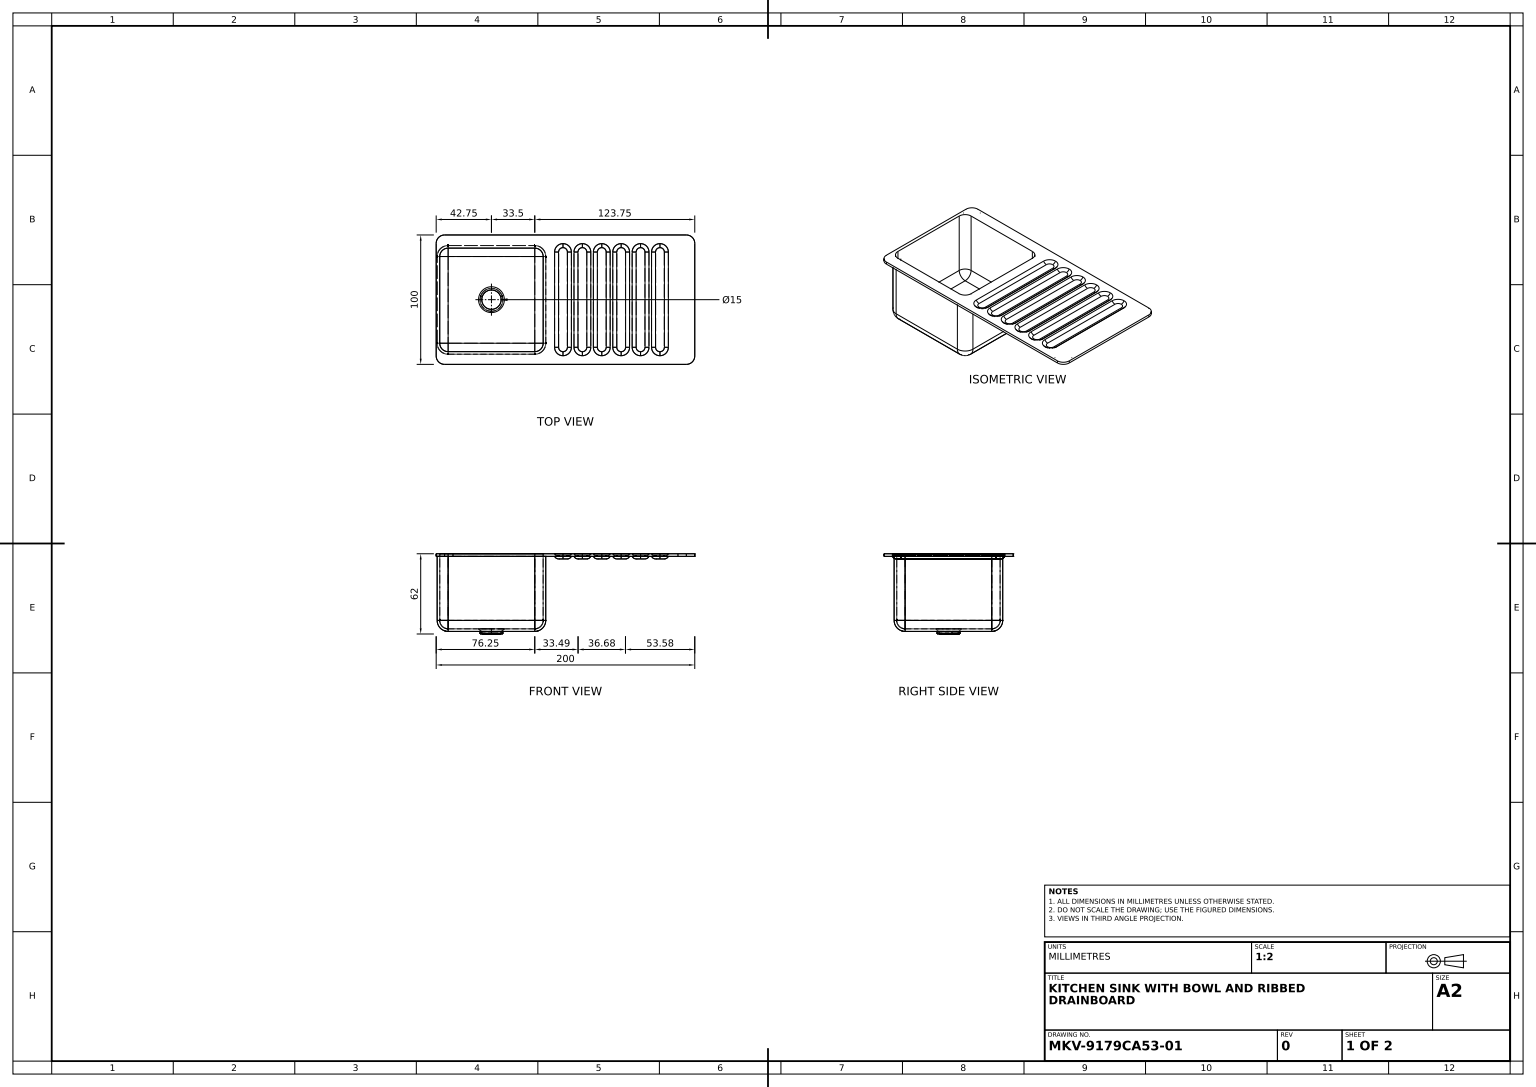
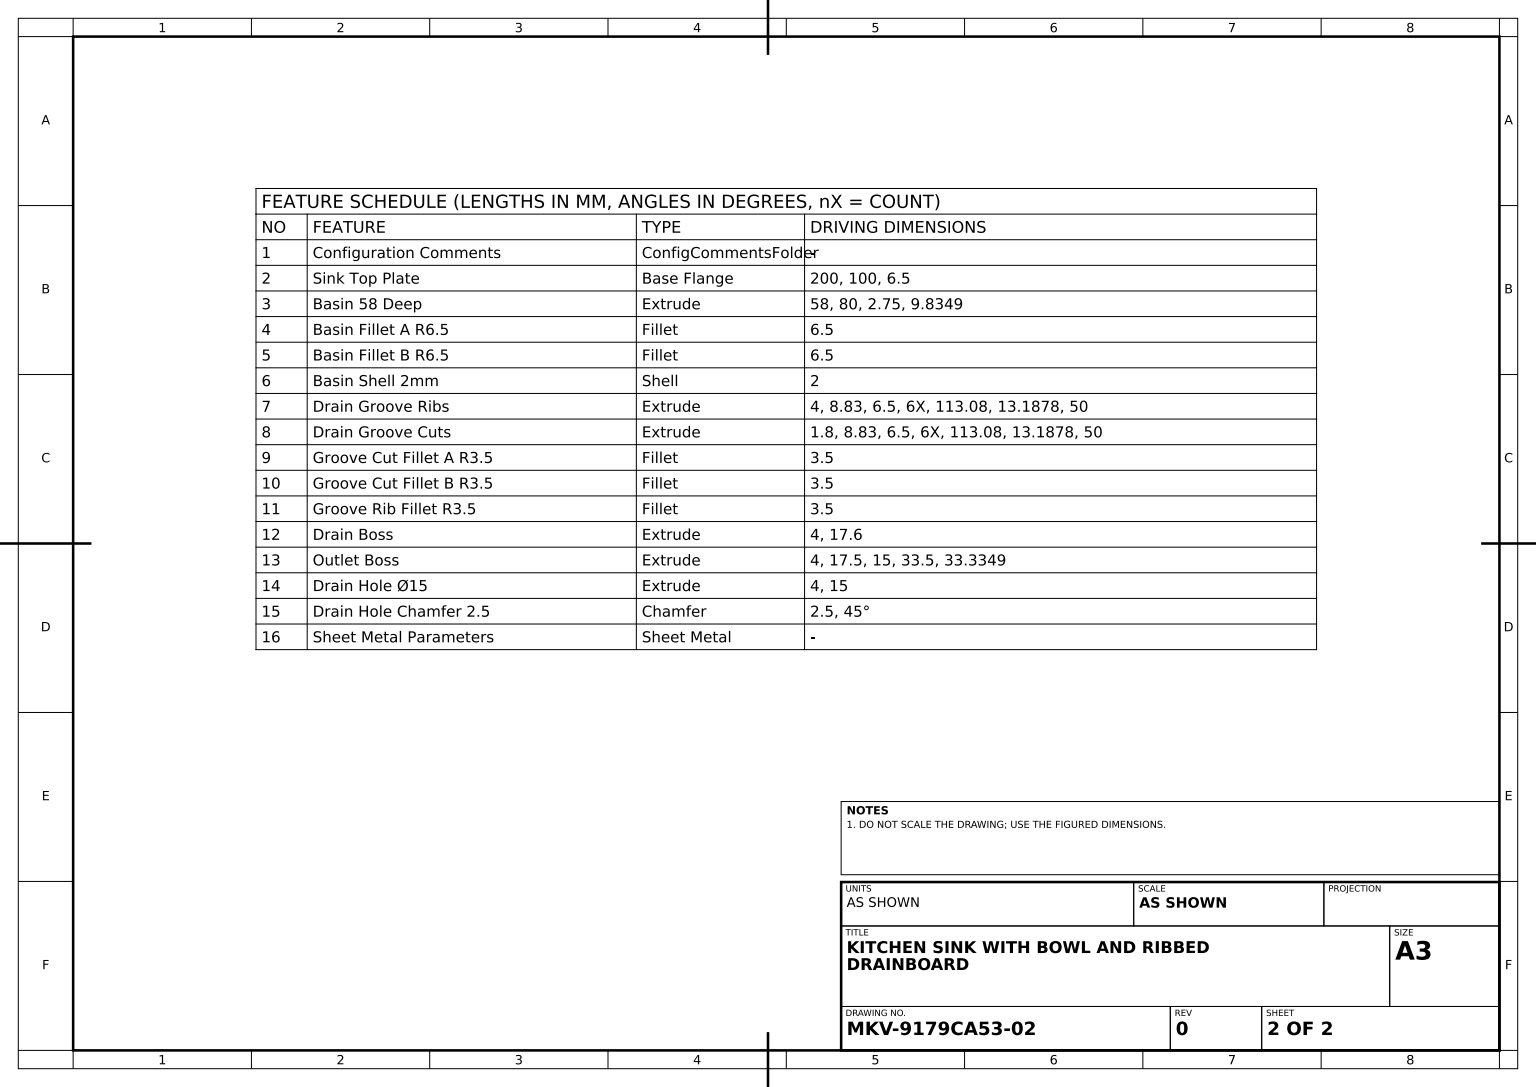
solid
v1 (16.520588,-1.8,36.8122)
v2 (19.58,0,36.8122)
e1 v1 v2 CIRCLE(AX(P(16.520588,1.7,36.8122),D(0,0,1),D(1,0,0)),3.5)
v3 (13.08,-1.8,40.252788)
e2 v3 v1 CIRCLE(AX(P(13.08,-1.8,36.8122),D(0,1,0),D(0,0,1)),3.440588)
v4 (13.08,0,43.3122)
e3 v4 v3 CIRCLE(AX(P(13.08,1.7,40.252788),D(1,0,0),D(0,0,-1)),3.5)
e4 v4 v2 CIRCLE(AX(P(13.08,0,36.8122),D(0,1,0),D(0,0,1)),6.5)
face TORUS(AX(P(13.08,1.7,36.8122),D(0,-1,0),D(0,0,-1)),3.440588,3.5) rev [-e1 -e2 -e3 e4]
v5 (9.742278,-4,36.8122)
v6 (6.58,-2,36.8122)
e5 v5 v6 CIRCLE(AX(P(9.742278,-0.5,36.8122),D(0,0,-1),D(-1,0,0)),3.5)
v7 (13.08,-4,40.149922)
e6 v7 v5 CIRCLE(AX(P(13.08,-4,36.8122),D(0,-1,0),D(0,0,1)),3.337722)
v8 (13.08,-2,43.3122)
e7 v8 v7 CIRCLE(AX(P(13.08,-0.5,40.149922),D(1,0,0),D(0,0,-1)),3.5)
e8 v8 v6 CIRCLE(AX(P(13.08,-2,36.8122),D(0,-1,0),D(0,0,-1)),6.5)
face TORUS(AX(P(13.08,-0.5,36.8122),D(0,-1,0),D(0,0,-1)),3.337722,3.5) [-e5 -e6 -e7 e8]
v9 (-90.75,-60,33.665098)
v10 (-23.75,-60,33.665098)
e9 v9 v10 LINE
v11 (-90.75,-60,-33.334902)
e10 v11 v9 LINE
v12 (-23.75,-60,-33.334902)
e11 v12 v11 LINE
e12 v10 v12 LINE
v13 (-48.887462,-60,-2.574969)
v14 (-57.25,-60,8.965098)
e13 v13 v14 CIRCLE(AX(P(-57.25,-60,0.165098),D(0,-1,0),D(0,0,-1)),8.8)
v15 (-65.612538,-60,-2.574969)
e14 v15 v13 CIRCLE(AX(P(-57.25,-60,0),D(0,-1,0),D(0,0,-1)),8.75)
e15 v14 v15 CIRCLE(AX(P(-57.25,-60,0.165098),D(0,-1,0),D(0,0,-1)),8.8)
face PLANE(AX(P(0,-60,0),D(0,-1,0),D(0,0,-1))) [-e9 -e10 -e11 -e12] [-e13 -e14 -e15]
v16 (-1.92,-1.8,40.252788)
v17 (1.520588,-1.8,36.8122)
e16 v16 v17 CIRCLE(AX(P(-1.92,-1.8,36.8122),D(0,1,0),D(0,0,1)),3.440588)
v18 (1.520588,-1.8,-36.8122)
e17 v17 v18 LINE
v19 (-1.92,-1.8,-40.252788)
e18 v18 v19 CIRCLE(AX(P(-1.92,-1.8,-36.8122),D(0,1,0),D(0,0,1)),3.440588)
v20 (-5.360588,-1.8,-36.8122)
e19 v19 v20 CIRCLE(AX(P(-1.92,-1.8,-36.8122),D(0,1,0),D(0,0,1)),3.440588)
v21 (-5.360588,-1.8,36.8122)
e20 v20 v21 LINE
e21 v21 v16 CIRCLE(AX(P(-1.92,-1.8,36.8122),D(0,1,0),D(0,0,1)),3.440588)
face PLANE(AX(P(-1.92,-1.8,-36.8122),D(0,1,0),D(0,0,1))) [e16 e17 e18 e19 e20 e21]
v22 (9.639412,-1.8,-36.8122)
v23 (9.639412,-1.8,36.8122)
e22 v22 v23 LINE
v24 (6.58,0,-36.8122)
e23 v24 v22 CIRCLE(AX(P(9.639412,1.7,-36.8122),D(0,0,1),D(1,0,0)),3.5)
v25 (6.58,0,36.8122)
e24 v24 v25 LINE
e25 v23 v25 CIRCLE(AX(P(9.639412,1.7,36.8122),D(0,0,-1),D(-1,0,0)),3.5)
face CYL(AX(P(9.639412,1.7,-36.8122),D(0,0,1),D(1,0,0)),3.5) rev [-e22 -e23 e24 -e25]
v26 (58.08,0,-43.3122)
v27 (58.08,-1.8,-40.252788)
e26 v26 v27 CIRCLE(AX(P(58.08,1.7,-40.252788),D(-1,0,0),D(0,0,1)),3.5)
v28 (51.58,0,-36.8122)
e27 v26 v28 CIRCLE(AX(P(58.08,0,-36.8122),D(0,1,0),D(0,0,1)),6.5)
v29 (54.639412,-1.8,-36.8122)
e28 v28 v29 CIRCLE(AX(P(54.639412,1.7,-36.8122),D(0,0,1),D(1,0,0)),3.5)
e29 v27 v29 CIRCLE(AX(P(58.08,-1.8,-36.8122),D(0,1,0),D(0,0,1)),3.440588)
face TORUS(AX(P(58.08,1.7,-36.8122),D(0,-1,0),D(0,0,-1)),3.440588,3.5) rev [-e26 e27 e28 -e29]
v30 (61.417722,-4,-36.8122)
v31 (61.417722,-4,36.8122)
e30 v30 v31 LINE
v32 (58.08,-4,40.149922)
e31 v31 v32 CIRCLE(AX(P(58.08,-4,36.8122),D(0,-1,0),D(0,0,1)),3.337722)
v33 (54.742278,-4,36.8122)
e32 v32 v33 CIRCLE(AX(P(58.08,-4,36.8122),D(0,-1,0),D(0,0,1)),3.337722)
v34 (54.742278,-4,-36.8122)
e33 v33 v34 LINE
v35 (58.08,-4,-40.149922)
e34 v34 v35 CIRCLE(AX(P(58.08,-4,-36.8122),D(0,-1,0),D(0,0,1)),3.337722)
e35 v35 v30 CIRCLE(AX(P(58.08,-4,-36.8122),D(0,-1,0),D(0,0,1)),3.337722)
face PLANE(AX(P(58.08,-4,-36.8122),D(0,1,0),D(0,0,1))) rev [e30 e31 e32 e33 e34 e35]
v36 (-93.5,0,-50)
v37 (-100,0,-43.5)
e36 v36 v37 CIRCLE(AX(P(-93.5,0,-43.5),D(0,1,0),D(0,0,-1)),6.5)
v38 (-93.5,-2,-50)
e37 v38 v36 LINE
v39 (-100,-2,-43.5)
e38 v38 v39 CIRCLE(AX(P(-93.5,-2,-43.5),D(0,1,0),D(0,0,-1)),6.5)
e39 v39 v37 LINE
face CYL(AX(P(-93.5,-60,-43.5),D(0,1,0),D(0,0,1)),6.5) [-e36 -e37 e38 e39]
v40 (51.58,0,36.8122)
v41 (58.08,0,43.3122)
e40 v40 v41 CIRCLE(AX(P(58.08,0,36.8122),D(0,1,0),D(0,0,1)),6.5)
v42 (58.08,-1.8,40.252788)
e41 v41 v42 CIRCLE(AX(P(58.08,1.7,40.252788),D(1,0,0),D(0,0,-1)),3.5)
v43 (54.639412,-1.8,36.8122)
e42 v43 v42 CIRCLE(AX(P(58.08,-1.8,36.8122),D(0,1,0),D(0,0,1)),3.440588)
e43 v43 v40 CIRCLE(AX(P(54.639412,1.7,36.8122),D(0,0,-1),D(-1,0,0)),3.5)
face TORUS(AX(P(58.08,1.7,36.8122),D(0,-1,0),D(0,0,-1)),3.440588,3.5) rev [e40 e41 -e42 e43]
v44 (-17.25,-51.5,33.665098)
v45 (-17.25,0,33.665098)
e44 v44 v45 LINE
v46 (-23.75,-51.5,40.165098)
e45 v46 v44 CIRCLE(AX(P(-23.75,-51.5,33.665098),D(0,1,0),D(0,0,1)),6.5)
v47 (-23.75,0,40.165098)
e46 v47 v46 LINE
e47 v45 v47 CIRCLE(AX(P(-23.75,0,33.665098),D(0,-1,0),D(0,0,-1)),6.5)
face CYL(AX(P(-23.75,-58,33.665098),D(0,-1,0),D(0,0,-1)),6.5) rev [-e44 -e45 -e46 -e47]
v48 (6.58,-2,-36.8122)
v49 (9.742278,-4,-36.8122)
e48 v48 v49 CIRCLE(AX(P(9.742278,-0.5,-36.8122),D(0,0,1),D(1,0,0)),3.5)
e49 v5 v49 LINE
e50 v6 v48 LINE
face CYL(AX(P(9.742278,-0.5,-36.8122),D(0,0,1),D(1,0,0)),3.5) [e48 -e49 e5 e50]
v50 (-15.25,-2,33.665098)
v51 (-15.25,-2,-33.334902)
e51 v50 v51 LINE
v52 (-15.25,-51.5,33.665098)
e52 v52 v50 LINE
v53 (-15.25,-51.5,-33.334902)
e53 v53 v52 LINE
e54 v51 v53 LINE
face PLANE(AX(P(-15.25,-58,40.165098),D(1,0,0),D(0,0,-1))) [-e51 -e52 -e53 -e54]
v54 (-5.257722,-4,-36.8122)
v55 (-1.92,-4,-40.149922)
e55 v54 v55 CIRCLE(AX(P(-1.92,-4,-36.8122),D(0,-1,0),D(0,0,1)),3.337722)
v56 (1.417722,-4,-36.8122)
e56 v55 v56 CIRCLE(AX(P(-1.92,-4,-36.8122),D(0,-1,0),D(0,0,1)),3.337722)
v57 (1.417722,-4,36.8122)
e57 v56 v57 LINE
v58 (-1.92,-4,40.149922)
e58 v57 v58 CIRCLE(AX(P(-1.92,-4,36.8122),D(0,-1,0),D(0,0,1)),3.337722)
v59 (-5.257722,-4,36.8122)
e59 v58 v59 CIRCLE(AX(P(-1.92,-4,36.8122),D(0,-1,0),D(0,0,1)),3.337722)
e60 v59 v54 LINE
face PLANE(AX(P(-1.92,-4,-36.8122),D(0,1,0),D(0,0,1))) rev [e55 e56 e57 e58 e59 e60]
v60 (66.58,0,-36.8122)
v61 (69.639412,-1.8,-36.8122)
e61 v60 v61 CIRCLE(AX(P(69.639412,1.7,-36.8122),D(0,0,1),D(1,0,0)),3.5)
v62 (66.58,0,36.8122)
e62 v60 v62 LINE
v63 (69.639412,-1.8,36.8122)
e63 v63 v62 CIRCLE(AX(P(69.639412,1.7,36.8122),D(0,0,-1),D(-1,0,0)),3.5)
e64 v61 v63 LINE
face CYL(AX(P(69.639412,1.7,-36.8122),D(0,0,1),D(1,0,0)),3.5) rev [-e61 e62 -e63 -e64]
v64 (24.639412,-1.8,36.8122)
v65 (21.58,0,36.8122)
e65 v64 v65 CIRCLE(AX(P(24.639412,1.7,36.8122),D(0,0,-1),D(-1,0,0)),3.5)
v66 (24.639412,-1.8,-36.8122)
e66 v66 v64 LINE
v67 (21.58,0,-36.8122)
e67 v67 v66 CIRCLE(AX(P(24.639412,1.7,-36.8122),D(0,0,1),D(1,0,0)),3.5)
e68 v67 v65 LINE
face CYL(AX(P(24.639412,1.7,-36.8122),D(0,0,1),D(1,0,0)),3.5) rev [-e65 -e66 -e67 e68]
v68 (-8.42,-2,-36.8122)
v69 (-1.92,-2,-43.3122)
e69 v68 v69 CIRCLE(AX(P(-1.92,-2,-36.8122),D(0,-1,0),D(0,0,-1)),6.5)
e70 v69 v55 CIRCLE(AX(P(-1.92,-0.5,-40.149922),D(-1,0,0),D(0,0,1)),3.5)
e71 v68 v54 CIRCLE(AX(P(-5.257722,-0.5,-36.8122),D(0,0,1),D(1,0,0)),3.5)
face TORUS(AX(P(-1.92,-0.5,-36.8122),D(0,-1,0),D(0,0,-1)),3.337722,3.5) [e69 e70 -e55 -e71]
v70 (64.58,-2,36.8122)
v71 (58.08,-2,43.3122)
e72 v70 v71 CIRCLE(AX(P(58.08,-2,36.8122),D(0,-1,0),D(0,0,-1)),6.5)
e73 v71 v32 CIRCLE(AX(P(58.08,-0.5,40.149922),D(1,0,0),D(0,0,-1)),3.5)
e74 v31 v70 CIRCLE(AX(P(61.417722,-0.5,36.8122),D(0,0,1),D(1,0,0)),3.5)
face TORUS(AX(P(58.08,-0.5,36.8122),D(0,-1,0),D(0,0,-1)),3.337722,3.5) [e72 e73 -e31 e74]
v72 (76.417722,-4,36.8122)
v73 (73.08,-4,40.149922)
e75 v72 v73 CIRCLE(AX(P(73.08,-4,36.8122),D(0,-1,0),D(0,0,1)),3.337722)
v74 (69.742278,-4,36.8122)
e76 v73 v74 CIRCLE(AX(P(73.08,-4,36.8122),D(0,-1,0),D(0,0,1)),3.337722)
v75 (69.742278,-4,-36.8122)
e77 v74 v75 LINE
v76 (73.08,-4,-40.149922)
e78 v75 v76 CIRCLE(AX(P(73.08,-4,-36.8122),D(0,-1,0),D(0,0,1)),3.337722)
v77 (76.417722,-4,-36.8122)
e79 v76 v77 CIRCLE(AX(P(73.08,-4,-36.8122),D(0,-1,0),D(0,0,1)),3.337722)
e80 v77 v72 LINE
face PLANE(AX(P(73.08,-4,-36.8122),D(0,1,0),D(0,0,1))) rev [e75 e76 e77 e78 e79 e80]
v78 (39.639412,-1.8,36.8122)
v79 (43.08,-1.8,40.252788)
e81 v78 v79 CIRCLE(AX(P(43.08,-1.8,36.8122),D(0,1,0),D(0,0,1)),3.440588)
v80 (36.58,0,36.8122)
e82 v78 v80 CIRCLE(AX(P(39.639412,1.7,36.8122),D(0,0,-1),D(-1,0,0)),3.5)
v81 (43.08,0,43.3122)
e83 v80 v81 CIRCLE(AX(P(43.08,0,36.8122),D(0,1,0),D(0,0,1)),6.5)
e84 v81 v79 CIRCLE(AX(P(43.08,1.7,40.252788),D(1,0,0),D(0,0,-1)),3.5)
face TORUS(AX(P(43.08,1.7,36.8122),D(0,-1,0),D(0,0,-1)),3.440588,3.5) rev [-e81 e82 e83 e84]
v82 (79.58,-2,36.8122)
e85 v72 v82 CIRCLE(AX(P(76.417722,-0.5,36.8122),D(0,0,1),D(1,0,0)),3.5)
v83 (79.58,-2,-36.8122)
e86 v83 v77 CIRCLE(AX(P(76.417722,-0.5,-36.8122),D(0,0,-1),D(-1,0,0)),3.5)
e87 v83 v82 LINE
face CYL(AX(P(76.417722,-0.5,-36.8122),D(0,0,-1),D(-1,0,0)),3.5) [-e85 -e80 -e86 e87]
v84 (-90.75,-2,42.165098)
v85 (-99.25,-2,33.665098)
e88 v84 v85 CIRCLE(AX(P(-90.75,-2,33.665098),D(0,-1,0),D(0,0,-1)),8.5)
v86 (-99.25,-51.5,33.665098)
e89 v85 v86 LINE
v87 (-90.75,-51.5,42.165098)
e90 v86 v87 CIRCLE(AX(P(-90.75,-51.5,33.665098),D(0,1,0),D(-1,0,0)),8.5)
e91 v87 v84 LINE
face CYL(AX(P(-90.75,-58,33.665098),D(0,1,0),D(0,0,1)),8.5) [e88 e89 e90 e91]
v88 (-90.75,-2,-41.834902)
v89 (-90.75,-51.5,-41.834902)
e92 v88 v89 LINE
v90 (-23.75,-2,-41.834902)
e93 v88 v90 LINE
v91 (-23.75,-51.5,-41.834902)
e94 v91 v90 LINE
e95 v89 v91 LINE
face PLANE(AX(P(-97.25,-58,-41.834902),D(0,0,1),D(1,0,0))) rev [-e92 e93 -e94 -e95]
v92 (-23.75,-2,42.165098)
v93 (-23.75,-51.5,42.165098)
e96 v92 v93 LINE
e97 v93 v52 CIRCLE(AX(P(-23.75,-51.5,33.665098),D(0,1,0),D(0,0,-1)),8.5)
e98 v50 v92 CIRCLE(AX(P(-23.75,-2,33.665098),D(0,-1,0),D(0,0,-1)),8.5)
face CYL(AX(P(-23.75,-58,33.665098),D(0,-1,0),D(0,0,-1)),8.5) [e96 e97 e52 e98]
v94 (39.742278,-4,-36.8122)
v95 (43.08,-4,-40.149922)
e99 v94 v95 CIRCLE(AX(P(43.08,-4,-36.8122),D(0,-1,0),D(0,0,1)),3.337722)
v96 (36.58,-2,-36.8122)
e100 v96 v94 CIRCLE(AX(P(39.742278,-0.5,-36.8122),D(0,0,1),D(1,0,0)),3.5)
v97 (43.08,-2,-43.3122)
e101 v96 v97 CIRCLE(AX(P(43.08,-2,-36.8122),D(0,-1,0),D(0,0,-1)),6.5)
e102 v97 v95 CIRCLE(AX(P(43.08,-0.5,-40.149922),D(-1,0,0),D(0,0,1)),3.5)
face TORUS(AX(P(43.08,-0.5,-36.8122),D(0,-1,0),D(0,0,-1)),3.337722,3.5) [-e99 -e100 e101 e102]
v98 (64.58,-2,-36.8122)
e103 v98 v30 CIRCLE(AX(P(61.417722,-0.5,-36.8122),D(0,0,-1),D(-1,0,0)),3.5)
e104 v98 v70 LINE
face CYL(AX(P(61.417722,-0.5,-36.8122),D(0,0,-1),D(-1,0,0)),3.5) [-e74 -e30 -e103 e104]
v99 (34.58,0,-36.8122)
v100 (28.08,0,-43.3122)
e105 v99 v100 CIRCLE(AX(P(28.08,0,-36.8122),D(0,1,0),D(0,0,1)),6.5)
v101 (28.08,-1.8,-40.252788)
e106 v100 v101 CIRCLE(AX(P(28.08,1.7,-40.252788),D(-1,0,0),D(0,0,1)),3.5)
v102 (31.520588,-1.8,-36.8122)
e107 v102 v101 CIRCLE(AX(P(28.08,-1.8,-36.8122),D(0,1,0),D(0,0,1)),3.440588)
e108 v99 v102 CIRCLE(AX(P(31.520588,1.7,-36.8122),D(0,0,-1),D(-1,0,0)),3.5)
face TORUS(AX(P(28.08,1.7,-36.8122),D(0,-1,0),D(0,0,-1)),3.440588,3.5) rev [e105 e106 -e107 -e108]
v103 (-99.25,-2,-33.334902)
e109 v103 v88 CIRCLE(AX(P(-90.75,-2,-33.334902),D(0,-1,0),D(0,0,-1)),8.5)
v104 (-99.25,-51.5,-33.334902)
e110 v89 v104 CIRCLE(AX(P(-90.75,-51.5,-33.334902),D(0,1,0),D(-1,0,0)),8.5)
e111 v104 v103 LINE
face CYL(AX(P(-90.75,-58,-33.334902),D(0,-1,0),D(0,0,-1)),8.5) [e109 e92 e110 e111]
v105 (73.08,-2,43.3122)
e112 v82 v105 CIRCLE(AX(P(73.08,-2,36.8122),D(0,-1,0),D(0,0,-1)),6.5)
e113 v105 v73 CIRCLE(AX(P(73.08,-0.5,40.149922),D(1,0,0),D(0,0,-1)),3.5)
face TORUS(AX(P(73.08,-0.5,36.8122),D(0,-1,0),D(0,0,-1)),3.337722,3.5) [e112 e113 -e75 e85]
v106 (-100,-2,43.5)
v107 (-100,0,43.5)
e114 v106 v107 LINE
e115 v37 v107 LINE
e116 v39 v106 LINE
face PLANE(AX(P(-100,-60,43.5),D(-1,0,0),D(0,0,1))) [e114 -e115 -e39 e116]
v108 (73.08,0,43.3122)
v109 (73.08,-1.8,40.252788)
e117 v108 v109 CIRCLE(AX(P(73.08,1.7,40.252788),D(1,0,0),D(0,0,-1)),3.5)
v110 (79.58,0,36.8122)
e118 v108 v110 CIRCLE(AX(P(73.08,0,36.8122),D(0,1,0),D(0,0,1)),6.5)
v111 (76.520588,-1.8,36.8122)
e119 v111 v110 CIRCLE(AX(P(76.520588,1.7,36.8122),D(0,0,1),D(1,0,0)),3.5)
e120 v109 v111 CIRCLE(AX(P(73.08,-1.8,36.8122),D(0,1,0),D(0,0,1)),3.440588)
face TORUS(AX(P(73.08,1.7,36.8122),D(0,-1,0),D(0,0,-1)),3.440588,3.5) rev [-e117 e118 -e119 -e120]
v112 (-90.75,-51.5,40.165098)
v113 (-90.75,0,40.165098)
e121 v112 v113 LINE
e122 v113 v47 LINE
e123 v46 v112 LINE
face PLANE(AX(P(-97.25,-58,40.165098),D(0,0,1),D(1,0,0))) rev [e121 e122 e46 e123]
v114 (-8.42,0,36.8122)
e124 v21 v114 CIRCLE(AX(P(-5.360588,1.7,36.8122),D(0,0,-1),D(-1,0,0)),3.5)
v115 (-1.92,0,43.3122)
e125 v114 v115 CIRCLE(AX(P(-1.92,0,36.8122),D(0,1,0),D(0,0,1)),6.5)
e126 v115 v16 CIRCLE(AX(P(-1.92,1.7,40.252788),D(1,0,0),D(0,0,-1)),3.5)
face TORUS(AX(P(-1.92,1.7,36.8122),D(0,-1,0),D(0,0,-1)),3.440588,3.5) rev [e124 e125 e126 -e21]
e127 v90 v51 CIRCLE(AX(P(-23.75,-2,-33.334902),D(0,-1,0),D(0,0,-1)),8.5)
e128 v53 v91 CIRCLE(AX(P(-23.75,-51.5,-33.334902),D(0,1,0),D(0,0,-1)),8.5)
face CYL(AX(P(-23.75,-58,-33.334902),D(0,1,0),D(0,0,1)),8.5) [e94 e127 e54 e128]
v116 (43.08,0,-43.3122)
v117 (43.08,-1.8,-40.252788)
e129 v116 v117 CIRCLE(AX(P(43.08,1.7,-40.252788),D(-1,0,0),D(0,0,1)),3.5)
v118 (36.58,0,-36.8122)
e130 v116 v118 CIRCLE(AX(P(43.08,0,-36.8122),D(0,1,0),D(0,0,1)),6.5)
v119 (39.639412,-1.8,-36.8122)
e131 v118 v119 CIRCLE(AX(P(39.639412,1.7,-36.8122),D(0,0,1),D(1,0,0)),3.5)
e132 v117 v119 CIRCLE(AX(P(43.08,-1.8,-36.8122),D(0,1,0),D(0,0,1)),3.440588)
face TORUS(AX(P(43.08,1.7,-36.8122),D(0,-1,0),D(0,0,-1)),3.440588,3.5) rev [-e129 e130 e131 -e132]
v120 (49.58,0,-36.8122)
v121 (46.520588,-1.8,-36.8122)
e133 v120 v121 CIRCLE(AX(P(46.520588,1.7,-36.8122),D(0,0,-1),D(-1,0,0)),3.5)
v122 (46.520588,-1.8,36.8122)
e134 v122 v121 LINE
v123 (49.58,0,36.8122)
e135 v122 v123 CIRCLE(AX(P(46.520588,1.7,36.8122),D(0,0,1),D(1,0,0)),3.5)
e136 v123 v120 LINE
face CYL(AX(P(46.520588,1.7,-36.8122),D(0,0,-1),D(-1,0,0)),3.5) rev [e133 -e134 e135 e136]
e137 v119 v78 LINE
e138 v79 v122 CIRCLE(AX(P(43.08,-1.8,36.8122),D(0,1,0),D(0,0,1)),3.440588)
e139 v121 v117 CIRCLE(AX(P(43.08,-1.8,-36.8122),D(0,1,0),D(0,0,1)),3.440588)
face PLANE(AX(P(43.08,-1.8,-36.8122),D(0,1,0),D(0,0,1))) [e132 e137 e81 e138 e134 e139]
v124 (16.520588,-1.8,-36.8122)
e140 v1 v124 LINE
v125 (19.58,0,-36.8122)
e141 v2 v125 LINE
e142 v125 v124 CIRCLE(AX(P(16.520588,1.7,-36.8122),D(0,0,-1),D(-1,0,0)),3.5)
face CYL(AX(P(16.520588,1.7,-36.8122),D(0,0,-1),D(-1,0,0)),3.5) rev [-e140 e1 e141 e142]
e143 v86 v9 CIRCLE(AX(P(-90.75,-51.5,33.665098),D(0,0,1),D(-1,0,0)),8.5)
e144 v86 v104 LINE
e145 v11 v104 CIRCLE(AX(P(-90.75,-51.5,-33.334902),D(0,0,-1),D(-1,0,0)),8.5)
face CYL(AX(P(-90.75,-51.5,40.165098),D(0,0,-1),D(-1,0,0)),8.5) [e10 -e143 e144 -e145]
v126 (19.58,-2,-36.8122)
v127 (16.417722,-4,-36.8122)
e146 v126 v127 CIRCLE(AX(P(16.417722,-0.5,-36.8122),D(0,0,-1),D(-1,0,0)),3.5)
v128 (13.08,-4,-40.149922)
e147 v128 v127 CIRCLE(AX(P(13.08,-4,-36.8122),D(0,-1,0),D(0,0,1)),3.337722)
v129 (13.08,-2,-43.3122)
e148 v129 v128 CIRCLE(AX(P(13.08,-0.5,-40.149922),D(-1,0,0),D(0,0,1)),3.5)
e149 v129 v126 CIRCLE(AX(P(13.08,-2,-36.8122),D(0,-1,0),D(0,0,-1)),6.5)
face TORUS(AX(P(13.08,-0.5,-36.8122),D(0,-1,0),D(0,0,-1)),3.337722,3.5) [e146 -e147 -e148 e149]
v130 (4.58,0,36.8122)
e150 v115 v130 CIRCLE(AX(P(-1.92,0,36.8122),D(0,1,0),D(0,0,1)),6.5)
e151 v17 v130 CIRCLE(AX(P(1.520588,1.7,36.8122),D(0,0,1),D(1,0,0)),3.5)
face TORUS(AX(P(-1.92,1.7,36.8122),D(0,-1,0),D(0,0,-1)),3.440588,3.5) rev [e150 -e151 -e16 -e126]
v131 (61.520588,-1.8,36.8122)
e152 v42 v131 CIRCLE(AX(P(58.08,-1.8,36.8122),D(0,1,0),D(0,0,1)),3.440588)
v132 (64.58,0,36.8122)
e153 v41 v132 CIRCLE(AX(P(58.08,0,36.8122),D(0,1,0),D(0,0,1)),6.5)
e154 v131 v132 CIRCLE(AX(P(61.520588,1.7,36.8122),D(0,0,1),D(1,0,0)),3.5)
face TORUS(AX(P(58.08,1.7,36.8122),D(0,-1,0),D(0,0,-1)),3.440588,3.5) rev [-e152 -e41 e153 -e154]
v133 (31.417722,-4,36.8122)
v134 (34.58,-2,36.8122)
e155 v133 v134 CIRCLE(AX(P(31.417722,-0.5,36.8122),D(0,0,1),D(1,0,0)),3.5)
v135 (28.08,-2,43.3122)
e156 v134 v135 CIRCLE(AX(P(28.08,-2,36.8122),D(0,-1,0),D(0,0,-1)),6.5)
v136 (28.08,-4,40.149922)
e157 v135 v136 CIRCLE(AX(P(28.08,-0.5,40.149922),D(1,0,0),D(0,0,-1)),3.5)
e158 v133 v136 CIRCLE(AX(P(28.08,-4,36.8122),D(0,-1,0),D(0,0,1)),3.337722)
face TORUS(AX(P(28.08,-0.5,36.8122),D(0,-1,0),D(0,0,-1)),3.337722,3.5) [e155 e156 e157 -e158]
v137 (51.58,-2,-36.8122)
e159 v137 v34 CIRCLE(AX(P(54.742278,-0.5,-36.8122),D(0,0,1),D(1,0,0)),3.5)
v138 (58.08,-2,-43.3122)
e160 v137 v138 CIRCLE(AX(P(58.08,-2,-36.8122),D(0,-1,0),D(0,0,-1)),6.5)
e161 v138 v35 CIRCLE(AX(P(58.08,-0.5,-40.149922),D(-1,0,0),D(0,0,1)),3.5)
face TORUS(AX(P(58.08,-0.5,-36.8122),D(0,-1,0),D(0,0,-1)),3.337722,3.5) [-e159 e160 e161 -e34]
e162 v100 v67 CIRCLE(AX(P(28.08,0,-36.8122),D(0,1,0),D(0,0,1)),6.5)
e163 v101 v66 CIRCLE(AX(P(28.08,-1.8,-36.8122),D(0,1,0),D(0,0,1)),3.440588)
face TORUS(AX(P(28.08,1.7,-36.8122),D(0,-1,0),D(0,0,-1)),3.440588,3.5) rev [-e106 e162 e67 -e163]
v139 (34.58,-2,-36.8122)
v140 (31.417722,-4,-36.8122)
e164 v139 v140 CIRCLE(AX(P(31.417722,-0.5,-36.8122),D(0,0,-1),D(-1,0,0)),3.5)
e165 v139 v134 LINE
e166 v140 v133 LINE
face CYL(AX(P(31.417722,-0.5,-36.8122),D(0,0,-1),D(-1,0,0)),3.5) [-e164 e165 -e155 -e166]
v141 (16.417722,-4,36.8122)
e167 v141 v7 CIRCLE(AX(P(13.08,-4,36.8122),D(0,-1,0),D(0,0,1)),3.337722)
v142 (19.58,-2,36.8122)
e168 v141 v142 CIRCLE(AX(P(16.417722,-0.5,36.8122),D(0,0,1),D(1,0,0)),3.5)
e169 v142 v8 CIRCLE(AX(P(13.08,-2,36.8122),D(0,-1,0),D(0,0,-1)),6.5)
face TORUS(AX(P(13.08,-0.5,36.8122),D(0,-1,0),D(0,0,-1)),3.337722,3.5) [e7 -e167 e168 e169]
v143 (-90.75,-51.5,-39.834902)
v144 (-97.25,-51.5,-33.334902)
e170 v143 v144 CIRCLE(AX(P(-90.75,-51.5,-33.334902),D(0,1,0),D(0,0,1)),6.5)
v145 (-90.75,-58,-33.334902)
e171 v145 v144 CIRCLE(AX(P(-90.75,-51.5,-33.334902),D(0,0,-1),D(-1,0,0)),6.5)
e172 v143 v145 CIRCLE(AX(P(-90.75,-51.5,-33.334902),D(-1,0,0),D(0,0,-1)),6.5)
face SPHERE(AX(P(-90.75,-51.5,-33.334902),D(0,1,0),D(1,0,0)),6.5) rev [e170 -e171 -e172]
v146 (93.5,0,-50)
e173 v146 v36 LINE
v147 (93.5,-2,-50)
e174 v147 v146 LINE
e175 v147 v38 LINE
face PLANE(AX(P(-93.5,-60,-50),D(0,0,-1),D(-1,0,0))) [-e173 -e174 e175 e37]
v148 (-97.25,0,33.665098)
v149 (-97.25,-51.5,33.665098)
e176 v148 v149 LINE
e177 v113 v148 CIRCLE(AX(P(-90.75,0,33.665098),D(0,-1,0),D(0,0,-1)),6.5)
e178 v149 v112 CIRCLE(AX(P(-90.75,-51.5,33.665098),D(0,1,0),D(0,0,1)),6.5)
face CYL(AX(P(-90.75,-58,33.665098),D(0,1,0),D(0,0,1)),6.5) rev [-e176 -e177 -e121 -e178]
e179 v29 v43 LINE
e180 v28 v40 LINE
face CYL(AX(P(54.639412,1.7,-36.8122),D(0,0,1),D(1,0,0)),3.5) rev [-e179 -e28 e180 -e43]
e181 v53 v12 CIRCLE(AX(P(-23.75,-51.5,-33.334902),D(0,0,-1),D(1,0,0)),8.5)
e182 v10 v52 CIRCLE(AX(P(-23.75,-51.5,33.665098),D(0,0,1),D(1,0,0)),8.5)
face CYL(AX(P(-23.75,-51.5,0),D(0,0,1),D(1,0,0)),8.5) [-e181 e53 -e182 e12]
v150 (-17.25,0,-33.334902)
v151 (-17.25,-51.5,-33.334902)
e183 v150 v151 LINE
v152 (-23.75,0,-39.834902)
e184 v152 v150 CIRCLE(AX(P(-23.75,0,-33.334902),D(0,-1,0),D(0,0,-1)),6.5)
v153 (-23.75,-51.5,-39.834902)
e185 v153 v152 LINE
e186 v151 v153 CIRCLE(AX(P(-23.75,-51.5,-33.334902),D(0,1,0),D(0,0,1)),6.5)
face CYL(AX(P(-23.75,-58,-33.334902),D(0,1,0),D(0,0,1)),6.5) rev [-e183 -e184 -e185 -e186]
e187 v93 v10 CIRCLE(AX(P(-23.75,-51.5,33.665098),D(1,0,0),D(0,0,1)),8.5)
face SPHERE(AX(P(-23.75,-51.5,33.665098),D(0,1,0),D(1,0,0)),8.5) [-e97 e187 e182]
e188 v93 v87 LINE
e189 v9 v87 CIRCLE(AX(P(-90.75,-51.5,33.665098),D(-1,0,0),D(0,0,1)),8.5)
face CYL(AX(P(0,-51.5,33.665098),D(-1,0,0),D(0,0,1)),8.5) [-e187 e188 -e189 e9]
v154 (28.08,-1.8,40.252788)
e190 v64 v154 CIRCLE(AX(P(28.08,-1.8,36.8122),D(0,1,0),D(0,0,1)),3.440588)
v155 (31.520588,-1.8,36.8122)
e191 v154 v155 CIRCLE(AX(P(28.08,-1.8,36.8122),D(0,1,0),D(0,0,1)),3.440588)
e192 v155 v102 LINE
face PLANE(AX(P(28.08,-1.8,-36.8122),D(0,1,0),D(0,0,1))) [e190 e191 e192 e107 e163 e66]
v156 (-48.887462,-62,-2.574969)
e193 v13 v156 LINE
v157 (-57.25,-62,8.965098)
e194 v157 v14 LINE
e195 v157 v156 CIRCLE(AX(P(-57.25,-62,0.165098),D(0,1,0),D(0,0,1)),8.8)
face CYL(AX(P(-57.25,-62,0.165098),D(0,1,0),D(0,0,1)),8.8) [-e193 e13 -e194 e195]
v158 (64.58,0,-36.8122)
e196 v158 v26 CIRCLE(AX(P(58.08,0,-36.8122),D(0,1,0),D(0,0,1)),6.5)
v159 (61.520588,-1.8,-36.8122)
e197 v159 v27 CIRCLE(AX(P(58.08,-1.8,-36.8122),D(0,1,0),D(0,0,1)),3.440588)
e198 v158 v159 CIRCLE(AX(P(61.520588,1.7,-36.8122),D(0,0,-1),D(-1,0,0)),3.5)
face TORUS(AX(P(58.08,1.7,-36.8122),D(0,-1,0),D(0,0,-1)),3.440588,3.5) rev [e196 e26 -e197 -e198]
v160 (93.5,-2,50)
v161 (93.5,0,50)
e199 v160 v161 LINE
v162 (100,-2,43.5)
e200 v160 v162 CIRCLE(AX(P(93.5,-2,43.5),D(0,1,0),D(0,0,-1)),6.5)
v163 (100,0,43.5)
e201 v162 v163 LINE
e202 v161 v163 CIRCLE(AX(P(93.5,0,43.5),D(0,1,0),D(0,0,1)),6.5)
face CYL(AX(P(93.5,-60,43.5),D(0,1,0),D(0,0,1)),6.5) [-e199 e200 e201 -e202]
v164 (-65.612538,-62,-2.574969)
e203 v164 v15 LINE
e204 v156 v164 CIRCLE(AX(P(-57.25,-62,0),D(0,1,0),D(0,0,1)),8.75)
face CYL(AX(P(-57.25,-62,0),D(0,1,0),D(0,0,1)),8.75) [e203 e14 e193 e204]
v165 (51.58,-2,36.8122)
e205 v33 v165 CIRCLE(AX(P(54.742278,-0.5,36.8122),D(0,0,-1),D(-1,0,0)),3.5)
e206 v165 v137 LINE
face CYL(AX(P(54.742278,-0.5,-36.8122),D(0,0,1),D(1,0,0)),3.5) [e205 e206 e159 -e33]
e207 v131 v159 LINE
face PLANE(AX(P(58.08,-1.8,-36.8122),D(0,1,0),D(0,0,1))) [e197 e29 e179 e42 e152 e207]
v166 (28.08,-2,-43.3122)
e208 v166 v139 CIRCLE(AX(P(28.08,-2,-36.8122),D(0,-1,0),D(0,0,-1)),6.5)
v167 (28.08,-4,-40.149922)
e209 v167 v140 CIRCLE(AX(P(28.08,-4,-36.8122),D(0,-1,0),D(0,0,1)),3.337722)
e210 v166 v167 CIRCLE(AX(P(28.08,-0.5,-40.149922),D(-1,0,0),D(0,0,1)),3.5)
face TORUS(AX(P(28.08,-0.5,-36.8122),D(0,-1,0),D(0,0,-1)),3.337722,3.5) [e208 e164 -e209 -e210]
v168 (-57.25,-60.5,7.5)
v169 (-57.25,-62,7.5)
e211 v168 v169 LINE
v170 (-57.25,-60.5,-7.5)
e212 v168 v170 CIRCLE(AX(P(-57.25,-60.5,0),D(0,1,0),D(0,0,-1)),7.5)
v171 (-57.25,-62,-7.5)
e213 v170 v171 LINE
e214 v171 v169 CIRCLE(AX(P(-57.25,-62,0),D(0,-1,0),D(0,0,-1)),7.5)
face CYL(AX(P(-57.25,-58,0),D(0,-1,0),D(0,0,-1)),7.5) rev [-e211 e212 e213 e214]
v172 (4.58,-2,36.8122)
v173 (-1.92,-2,43.3122)
e215 v172 v173 CIRCLE(AX(P(-1.92,-2,36.8122),D(0,-1,0),D(0,0,-1)),6.5)
e216 v173 v58 CIRCLE(AX(P(-1.92,-0.5,40.149922),D(1,0,0),D(0,0,-1)),3.5)
e217 v57 v172 CIRCLE(AX(P(1.417722,-0.5,36.8122),D(0,0,1),D(1,0,0)),3.5)
face TORUS(AX(P(-1.92,-0.5,36.8122),D(0,-1,0),D(0,0,-1)),3.337722,3.5) [e215 e216 -e58 e217]
v174 (39.742278,-4,36.8122)
v175 (36.58,-2,36.8122)
e218 v174 v175 CIRCLE(AX(P(39.742278,-0.5,36.8122),D(0,0,-1),D(-1,0,0)),3.5)
e219 v175 v96 LINE
e220 v174 v94 LINE
face CYL(AX(P(39.742278,-0.5,-36.8122),D(0,0,1),D(1,0,0)),3.5) [e218 e219 e100 -e220]
v176 (-90.75,0,-39.834902)
e221 v176 v152 LINE
e222 v176 v143 LINE
e223 v143 v153 LINE
face PLANE(AX(P(-97.25,-58,-39.834902),D(0,0,1),D(1,0,0))) [e185 -e221 e222 e223]
v177 (66.58,-2,36.8122)
e224 v74 v177 CIRCLE(AX(P(69.742278,-0.5,36.8122),D(0,0,-1),D(-1,0,0)),3.5)
e225 v105 v177 CIRCLE(AX(P(73.08,-2,36.8122),D(0,-1,0),D(0,0,-1)),6.5)
face TORUS(AX(P(73.08,-0.5,36.8122),D(0,-1,0),D(0,0,-1)),3.337722,3.5) [-e224 -e76 -e113 e225]
v178 (66.58,-2,-36.8122)
e226 v178 v75 CIRCLE(AX(P(69.742278,-0.5,-36.8122),D(0,0,1),D(1,0,0)),3.5)
v179 (73.08,-2,-43.3122)
e227 v178 v179 CIRCLE(AX(P(73.08,-2,-36.8122),D(0,-1,0),D(0,0,-1)),6.5)
e228 v179 v76 CIRCLE(AX(P(73.08,-0.5,-40.149922),D(-1,0,0),D(0,0,1)),3.5)
face TORUS(AX(P(73.08,-0.5,-36.8122),D(0,-1,0),D(0,0,-1)),3.337722,3.5) [-e226 e227 e228 -e78]
v180 (13.08,-1.8,-40.252788)
e229 v124 v180 CIRCLE(AX(P(13.08,-1.8,-36.8122),D(0,1,0),D(0,0,1)),3.440588)
v181 (13.08,0,-43.3122)
e230 v125 v181 CIRCLE(AX(P(13.08,0,-36.8122),D(0,1,0),D(0,0,1)),6.5)
e231 v181 v180 CIRCLE(AX(P(13.08,1.7,-40.252788),D(-1,0,0),D(0,0,1)),3.5)
face TORUS(AX(P(13.08,1.7,-36.8122),D(0,-1,0),D(0,0,-1)),3.440588,3.5) rev [-e229 -e142 e230 e231]
e232 v177 v178 LINE
face CYL(AX(P(69.742278,-0.5,-36.8122),D(0,0,1),D(1,0,0)),3.5) [-e77 e224 e232 e226]
e233 v23 v3 CIRCLE(AX(P(13.08,-1.8,36.8122),D(0,1,0),D(0,0,1)),3.440588)
e234 v180 v22 CIRCLE(AX(P(13.08,-1.8,-36.8122),D(0,1,0),D(0,0,1)),3.440588)
face PLANE(AX(P(13.08,-1.8,-36.8122),D(0,1,0),D(0,0,1))) [e233 e2 e140 e229 e234 e22]
v182 (-93.5,-2,50)
v183 (-93.5,0,50)
e235 v182 v183 LINE
e236 v182 v160 LINE
e237 v183 v161 LINE
face PLANE(AX(P(-93.5,-60,50),D(0,0,1),D(1,0,0))) [-e235 e236 e199 -e237]
e238 v45 v150 LINE
e239 v151 v44 LINE
face PLANE(AX(P(-17.25,-58,40.165098),D(1,0,0),D(0,0,-1))) rev [e44 e238 e183 e239]
v184 (-1.92,0,-43.3122)
v185 (-8.42,0,-36.8122)
e240 v184 v185 CIRCLE(AX(P(-1.92,0,-36.8122),D(0,1,0),D(0,0,1)),6.5)
e241 v185 v20 CIRCLE(AX(P(-5.360588,1.7,-36.8122),D(0,0,1),D(1,0,0)),3.5)
e242 v184 v19 CIRCLE(AX(P(-1.92,1.7,-40.252788),D(-1,0,0),D(0,0,1)),3.5)
face TORUS(AX(P(-1.92,1.7,-36.8122),D(0,-1,0),D(0,0,-1)),3.440588,3.5) rev [e240 e241 -e19 -e242]
v186 (21.58,-2,36.8122)
e243 v135 v186 CIRCLE(AX(P(28.08,-2,36.8122),D(0,-1,0),D(0,0,-1)),6.5)
v187 (24.742278,-4,36.8122)
e244 v187 v186 CIRCLE(AX(P(24.742278,-0.5,36.8122),D(0,0,-1),D(-1,0,0)),3.5)
e245 v136 v187 CIRCLE(AX(P(28.08,-4,36.8122),D(0,-1,0),D(0,0,1)),3.337722)
face TORUS(AX(P(28.08,-0.5,36.8122),D(0,-1,0),D(0,0,-1)),3.337722,3.5) [-e157 e243 -e244 -e245]
v188 (49.58,-2,-36.8122)
e246 v97 v188 CIRCLE(AX(P(43.08,-2,-36.8122),D(0,-1,0),D(0,0,-1)),6.5)
v189 (46.417722,-4,-36.8122)
e247 v188 v189 CIRCLE(AX(P(46.417722,-0.5,-36.8122),D(0,0,-1),D(-1,0,0)),3.5)
e248 v95 v189 CIRCLE(AX(P(43.08,-4,-36.8122),D(0,-1,0),D(0,0,1)),3.337722)
face TORUS(AX(P(43.08,-0.5,-36.8122),D(0,-1,0),D(0,0,-1)),3.337722,3.5) [e246 e247 -e248 -e102]
v190 (46.417722,-4,36.8122)
e249 v189 v190 LINE
v191 (43.08,-4,40.149922)
e250 v190 v191 CIRCLE(AX(P(43.08,-4,36.8122),D(0,-1,0),D(0,0,1)),3.337722)
e251 v191 v174 CIRCLE(AX(P(43.08,-4,36.8122),D(0,-1,0),D(0,0,1)),3.337722)
face PLANE(AX(P(43.08,-4,-36.8122),D(0,1,0),D(0,0,1))) rev [e99 e248 e249 e250 e251 e220]
e252 v170 v168 CIRCLE(AX(P(-57.25,-60.5,0),D(0,1,0),D(0,0,-1)),7.5)
e253 v169 v171 CIRCLE(AX(P(-57.25,-62,0),D(0,-1,0),D(0,0,-1)),7.5)
face CYL(AX(P(-57.25,-58,0),D(0,-1,0),D(0,0,-1)),7.5) rev [e252 e211 e253 -e213]
e254 v84 v92 LINE
face PLANE(AX(P(-97.25,-58,42.165098),D(0,0,1),D(1,0,0))) [-e91 -e188 -e96 -e254]
v192 (34.58,0,36.8122)
e255 v192 v99 LINE
e256 v155 v192 CIRCLE(AX(P(31.520588,1.7,36.8122),D(0,0,1),D(1,0,0)),3.5)
face CYL(AX(P(31.520588,1.7,-36.8122),D(0,0,-1),D(-1,0,0)),3.5) rev [e255 e108 -e192 e256]
e257 v25 v4 CIRCLE(AX(P(13.08,0,36.8122),D(0,1,0),D(0,0,1)),6.5)
face TORUS(AX(P(13.08,1.7,36.8122),D(0,-1,0),D(0,0,-1)),3.440588,3.5) rev [e257 e3 -e233 e25]
e258 v81 v123 CIRCLE(AX(P(43.08,0,36.8122),D(0,1,0),D(0,0,1)),6.5)
face TORUS(AX(P(43.08,1.7,36.8122),D(0,-1,0),D(0,0,-1)),3.440588,3.5) rev [-e135 -e138 -e84 e258]
v193 (4.58,-2,-36.8122)
e259 v69 v193 CIRCLE(AX(P(-1.92,-2,-36.8122),D(0,-1,0),D(0,0,-1)),6.5)
e260 v193 v56 CIRCLE(AX(P(1.417722,-0.5,-36.8122),D(0,0,-1),D(-1,0,0)),3.5)
face TORUS(AX(P(-1.92,-0.5,-36.8122),D(0,-1,0),D(0,0,-1)),3.337722,3.5) [e259 e260 -e56 -e70]
v194 (24.742278,-4,-36.8122)
e261 v187 v194 LINE
e262 v194 v167 CIRCLE(AX(P(28.08,-4,-36.8122),D(0,-1,0),D(0,0,1)),3.337722)
face PLANE(AX(P(28.08,-4,-36.8122),D(0,1,0),D(0,0,1))) rev [e245 e261 e262 e209 e166 e158]
v195 (-57.25,-58,10)
e263 v168 v195 LINE
v196 (-57.25,-58,-10)
e264 v196 v195 CIRCLE(AX(P(-57.25,-58,0),D(0,-1,0),D(0,0,-1)),10)
e265 v170 v196 LINE
face CONE(AX(P(-57.25,-58,0),D(0,1,0),D(0,0,1)),10,0.785398163) rev [-e212 e263 -e264 -e265]
e266 v132 v158 LINE
face CYL(AX(P(61.520588,1.7,-36.8122),D(0,0,-1),D(-1,0,0)),3.5) rev [e198 -e207 e154 e266]
v197 (-97.25,0,-33.334902)
e267 v144 v197 LINE
e268 v197 v176 CIRCLE(AX(P(-90.75,0,-33.334902),D(0,-1,0),D(0,0,-1)),6.5)
face CYL(AX(P(-90.75,-58,-33.334902),D(0,-1,0),D(0,0,-1)),6.5) rev [-e267 -e170 -e222 -e268]
v198 (100,0,-43.5)
e269 v198 v146 CIRCLE(AX(P(93.5,0,-43.5),D(0,1,0),D(0,0,-1)),6.5)
v199 (100,-2,-43.5)
e270 v199 v198 LINE
e271 v199 v147 CIRCLE(AX(P(93.5,-2,-43.5),D(0,1,0),D(0,0,-1)),6.5)
face CYL(AX(P(93.5,-60,-43.5),D(0,1,0),D(0,0,1)),6.5) [e174 -e269 -e270 e271]
v200 (28.08,0,43.3122)
e272 v200 v192 CIRCLE(AX(P(28.08,0,36.8122),D(0,1,0),D(0,0,1)),6.5)
e273 v65 v200 CIRCLE(AX(P(28.08,0,36.8122),D(0,1,0),D(0,0,1)),6.5)
v201 (4.58,0,-36.8122)
e274 v130 v201 LINE
e275 v185 v114 LINE
e276 v201 v184 CIRCLE(AX(P(-1.92,0,-36.8122),D(0,1,0),D(0,0,1)),6.5)
e277 v163 v198 LINE
e278 v107 v183 CIRCLE(AX(P(-93.5,0,43.5),D(0,1,0),D(0,0,-1)),6.5)
e279 v120 v116 CIRCLE(AX(P(43.08,0,-36.8122),D(0,1,0),D(0,0,1)),6.5)
e280 v118 v80 LINE
e281 v148 v197 LINE
e282 v181 v24 CIRCLE(AX(P(13.08,0,-36.8122),D(0,1,0),D(0,0,1)),6.5)
v202 (79.58,0,-36.8122)
v203 (73.08,0,-43.3122)
e283 v202 v203 CIRCLE(AX(P(73.08,0,-36.8122),D(0,1,0),D(0,0,1)),6.5)
e284 v110 v202 LINE
e285 v62 v108 CIRCLE(AX(P(73.08,0,36.8122),D(0,1,0),D(0,0,1)),6.5)
e286 v203 v60 CIRCLE(AX(P(73.08,0,-36.8122),D(0,1,0),D(0,0,1)),6.5)
face PLANE(AX(P(93.5,0,-43.5),D(0,-1,0),D(0,0,-1))) rev [-e162 -e105 -e255 -e272 -e273 -e68] [-e274 -e150 -e125 -e275 -e240 -e276] [e202 e277 e269 e173 e36 e115 e278 e237] [-e130 -e279 -e136 -e258 -e83 -e280] [e281 e268 e221 e184 -e238 e47 -e122 e177] [-e40 -e180 -e27 -e196 -e266 -e153] [-e4 -e257 -e24 -e282 -e230 -e141] [-e283 -e284 -e118 -e285 -e62 -e286]
v204 (-8.42,-2,36.8122)
e287 v173 v204 CIRCLE(AX(P(-1.92,-2,36.8122),D(0,-1,0),D(0,0,-1)),6.5)
e288 v59 v204 CIRCLE(AX(P(-5.257722,-0.5,36.8122),D(0,0,-1),D(-1,0,0)),3.5)
face TORUS(AX(P(-1.92,-0.5,36.8122),D(0,-1,0),D(0,0,-1)),3.337722,3.5) [-e216 e287 -e288 -e59]
e289 v89 v11 CIRCLE(AX(P(-90.75,-51.5,-33.334902),D(-1,0,0),D(0,0,-1)),8.5)
face SPHERE(AX(P(-90.75,-51.5,-33.334902),D(0,1,0),D(1,0,0)),8.5) [-e110 e289 e145]
e290 v195 v196 CIRCLE(AX(P(-57.25,-58,0),D(0,-1,0),D(0,0,-1)),10)
face CONE(AX(P(-57.25,-58,0),D(0,1,0),D(0,0,1)),10,0.785398163) rev [-e290 -e263 -e252 e265]
v205 (76.520588,-1.8,-36.8122)
v206 (73.08,-1.8,-40.252788)
e291 v205 v206 CIRCLE(AX(P(73.08,-1.8,-36.8122),D(0,1,0),D(0,0,1)),3.440588)
e292 v202 v205 CIRCLE(AX(P(76.520588,1.7,-36.8122),D(0,0,-1),D(-1,0,0)),3.5)
e293 v203 v206 CIRCLE(AX(P(73.08,1.7,-40.252788),D(-1,0,0),D(0,0,1)),3.5)
face TORUS(AX(P(73.08,1.7,-36.8122),D(0,-1,0),D(0,0,-1)),3.440588,3.5) rev [-e291 -e292 e283 e293]
e294 v48 v129 CIRCLE(AX(P(13.08,-2,-36.8122),D(0,-1,0),D(0,0,-1)),6.5)
e295 v49 v128 CIRCLE(AX(P(13.08,-4,-36.8122),D(0,-1,0),D(0,0,1)),3.337722)
face TORUS(AX(P(13.08,-0.5,-36.8122),D(0,-1,0),D(0,0,-1)),3.337722,3.5) [-e48 e294 e148 -e295]
e296 v63 v109 CIRCLE(AX(P(73.08,-1.8,36.8122),D(0,1,0),D(0,0,1)),3.440588)
face TORUS(AX(P(73.08,1.7,36.8122),D(0,-1,0),D(0,0,-1)),3.440588,3.5) rev [e63 e285 e117 -e296]
e297 v111 v205 LINE
face CYL(AX(P(76.520588,1.7,-36.8122),D(0,0,-1),D(-1,0,0)),3.5) rev [e284 e292 -e297 e119]
v207 (49.58,-2,36.8122)
e298 v190 v207 CIRCLE(AX(P(46.417722,-0.5,36.8122),D(0,0,1),D(1,0,0)),3.5)
v208 (43.08,-2,43.3122)
e299 v207 v208 CIRCLE(AX(P(43.08,-2,36.8122),D(0,-1,0),D(0,0,-1)),6.5)
e300 v208 v191 CIRCLE(AX(P(43.08,-0.5,40.149922),D(1,0,0),D(0,0,-1)),3.5)
face TORUS(AX(P(43.08,-0.5,36.8122),D(0,-1,0),D(0,0,-1)),3.337722,3.5) [e298 e299 e300 -e250]
e301 v162 v199 LINE
face PLANE(AX(P(100,-60,43.5),D(1,0,0),D(0,0,-1))) [-e277 -e201 e301 e270]
e302 v206 v61 CIRCLE(AX(P(73.08,-1.8,-36.8122),D(0,1,0),D(0,0,1)),3.440588)
face TORUS(AX(P(73.08,1.7,-36.8122),D(0,-1,0),D(0,0,-1)),3.440588,3.5) rev [-e293 e286 e61 -e302]
v209 (-23.75,-58,33.665098)
e303 v46 v209 CIRCLE(AX(P(-23.75,-51.5,33.665098),D(1,0,0),D(0,0,1)),6.5)
v210 (-90.75,-58,33.665098)
e304 v210 v209 LINE
e305 v210 v112 CIRCLE(AX(P(-90.75,-51.5,33.665098),D(-1,0,0),D(0,0,1)),6.5)
face CYL(AX(P(0,-51.5,33.665098),D(-1,0,0),D(0,0,1)),6.5) rev [-e123 e303 -e304 e305]
e306 v12 v91 CIRCLE(AX(P(-23.75,-51.5,-33.334902),D(1,0,0),D(0,0,-1)),8.5)
face CYL(AX(P(-97.25,-51.5,-33.334902),D(1,0,0),D(0,0,-1)),8.5) [-e306 e11 -e289 e95]
e307 v188 v207 LINE
face CYL(AX(P(46.417722,-0.5,-36.8122),D(0,0,-1),D(-1,0,0)),3.5) [-e249 -e247 e307 -e298]
face TORUS(AX(P(13.08,1.7,-36.8122),D(0,-1,0),D(0,0,-1)),3.440588,3.5) rev [-e234 -e231 e282 e23]
v211 (-23.75,-58,-33.334902)
e308 v151 v211 CIRCLE(AX(P(-23.75,-51.5,-33.334902),D(0,0,-1),D(1,0,0)),6.5)
e309 v211 v153 CIRCLE(AX(P(-23.75,-51.5,-33.334902),D(1,0,0),D(0,0,-1)),6.5)
face SPHERE(AX(P(-23.75,-51.5,-33.334902),D(0,1,0),D(1,0,0)),6.5) rev [-e308 e186 -e309]
e310 v193 v172 LINE
face CYL(AX(P(1.417722,-0.5,-36.8122),D(0,0,-1),D(-1,0,0)),3.5) [e310 -e217 -e57 -e260]
e311 v201 v18 CIRCLE(AX(P(1.520588,1.7,-36.8122),D(0,0,-1),D(-1,0,0)),3.5)
face CYL(AX(P(1.520588,1.7,-36.8122),D(0,0,-1),D(-1,0,0)),3.5) rev [e311 -e17 e151 e274]
e312 v208 v175 CIRCLE(AX(P(43.08,-2,36.8122),D(0,-1,0),D(0,0,-1)),6.5)
face TORUS(AX(P(43.08,-0.5,36.8122),D(0,-1,0),D(0,0,-1)),3.337722,3.5) [-e300 e312 -e218 -e251]
e313 v71 v165 CIRCLE(AX(P(58.08,-2,36.8122),D(0,-1,0),D(0,0,-1)),6.5)
face TORUS(AX(P(58.08,-0.5,36.8122),D(0,-1,0),D(0,0,-1)),3.337722,3.5) [-e205 -e32 -e73 e313]
face CYL(AX(P(39.639412,1.7,-36.8122),D(0,0,1),D(1,0,0)),3.5) rev [e280 -e82 -e137 -e131]
e314 v204 v68 LINE
face CYL(AX(P(-5.257722,-0.5,-36.8122),D(0,0,1),D(1,0,0)),3.5) [e314 e71 -e60 e288]
face PLANE(AX(P(73.08,-1.8,-36.8122),D(0,1,0),D(0,0,1))) [e291 e302 e64 e296 e120 e297]
e315 v209 v44 CIRCLE(AX(P(-23.75,-51.5,33.665098),D(0,0,1),D(1,0,0)),6.5)
e316 v209 v211 LINE
face CYL(AX(P(-23.75,-51.5,0),D(0,0,1),D(1,0,0)),6.5) rev [e315 -e239 e308 -e316]
e317 v127 v141 LINE
e318 v126 v142 LINE
face CYL(AX(P(16.417722,-0.5,-36.8122),D(0,0,-1),D(-1,0,0)),3.5) [-e168 -e317 -e146 e318]
e319 v211 v145 LINE
face CYL(AX(P(-97.25,-51.5,-33.334902),D(1,0,0),D(0,0,-1)),6.5) rev [-e223 e172 -e319 e309]
e320 v85 v103 LINE
face PLANE(AX(P(-99.25,-58,40.165098),D(1,0,0),D(0,0,-1))) rev [e320 -e111 -e144 -e89]
face PLANE(AX(P(13.08,-4,-36.8122),D(0,1,0),D(0,0,1))) rev [e6 e49 e295 e147 e317 e167]
e321 v164 v157 CIRCLE(AX(P(-57.25,-62,0.165098),D(0,1,0),D(0,0,1)),8.8)
face PLANE(AX(P(-57.25,-62,0.165098),D(0,1,0),D(0,0,1))) rev [-e204 -e195 -e321] [-e253 -e214]
e322 v200 v154 CIRCLE(AX(P(28.08,1.7,40.252788),D(1,0,0),D(0,0,-1)),3.5)
face TORUS(AX(P(28.08,1.7,36.8122),D(0,-1,0),D(0,0,-1)),3.440588,3.5) rev [e272 -e256 -e191 -e322]
e323 v149 v144 LINE
face PLANE(AX(P(-97.25,-58,40.165098),D(1,0,0),D(0,0,-1))) [e176 e323 e267 -e281]
v212 (21.58,-2,-36.8122)
e324 v212 v194 CIRCLE(AX(P(24.742278,-0.5,-36.8122),D(0,0,1),D(1,0,0)),3.5)
e325 v212 v166 CIRCLE(AX(P(28.08,-2,-36.8122),D(0,-1,0),D(0,0,-1)),6.5)
face TORUS(AX(P(28.08,-0.5,-36.8122),D(0,-1,0),D(0,0,-1)),3.337722,3.5) [e210 -e262 -e324 e325]
face SPHERE(AX(P(-23.75,-51.5,33.665098),D(0,1,0),D(1,0,0)),6.5) rev [-e315 -e303 e45]
e326 v138 v98 CIRCLE(AX(P(58.08,-2,-36.8122),D(0,-1,0),D(0,0,-1)),6.5)
face TORUS(AX(P(58.08,-0.5,-36.8122),D(0,-1,0),D(0,0,-1)),3.337722,3.5) [-e161 e326 e103 -e35]
face CYL(AX(P(-5.360588,1.7,-36.8122),D(0,0,1),D(1,0,0)),3.5) rev [e275 -e124 -e20 -e241]
e327 v186 v212 LINE
e328 v179 v83 CIRCLE(AX(P(73.08,-2,-36.8122),D(0,-1,0),D(0,0,-1)),6.5)
e329 v106 v182 CIRCLE(AX(P(-93.5,-2,43.5),D(0,1,0),D(0,0,-1)),6.5)
face PLANE(AX(P(93.5,-2,-43.5),D(0,-1,0),D(0,0,-1))) [-e93 -e109 -e320 -e88 e254 -e98 e51 -e127] [-e208 -e325 -e327 -e243 -e156 -e165] [-e149 -e294 -e50 -e8 -e169 -e318] [-e69 -e314 -e287 -e215 -e310 -e259] [-e160 -e206 -e313 -e72 -e104 -e326] [-e219 -e312 -e299 -e307 -e246 -e101] [-e225 -e112 -e87 -e328 -e227 -e232] [-e236 -e329 -e116 -e38 -e175 -e271 -e301 -e200]
face CYL(AX(P(24.742278,-0.5,-36.8122),D(0,0,1),D(1,0,0)),3.5) [e244 e327 e324 -e261]
face CYL(AX(P(-93.5,-60,43.5),D(0,1,0),D(0,0,1)),6.5) [e235 -e278 -e114 e329]
face CYL(AX(P(-57.25,-62,0.165098),D(0,1,0),D(0,0,1)),8.8) [e194 e15 -e203 e321]
face TORUS(AX(P(43.08,1.7,-36.8122),D(0,-1,0),D(0,0,-1)),3.440588,3.5) rev [-e133 e279 e129 -e139]
face TORUS(AX(P(73.08,-0.5,-36.8122),D(0,-1,0),D(0,0,-1)),3.337722,3.5) [e86 -e79 -e228 e328]
face TORUS(AX(P(-1.92,1.7,-36.8122),D(0,-1,0),D(0,0,-1)),3.440588,3.5) rev [-e311 e276 e242 -e18]
e330 v149 v210 CIRCLE(AX(P(-90.75,-51.5,33.665098),D(0,0,1),D(-1,0,0)),6.5)
e331 v145 v210 LINE
face CYL(AX(P(-90.75,-51.5,40.165098),D(0,0,-1),D(-1,0,0)),6.5) rev [e171 -e323 e330 -e331]
face TORUS(AX(P(28.08,1.7,36.8122),D(0,-1,0),D(0,0,-1)),3.440588,3.5) rev [e322 -e190 e65 e273]
face SPHERE(AX(P(-90.75,-51.5,33.665098),D(0,1,0),D(1,0,0)),8.5) [e189 -e90 e143]
face PLANE(AX(P(0,-58,0),D(0,-1,0),D(0,0,-1))) rev [e290 e264] [e331 e304 e316 e319]
face SPHERE(AX(P(-90.75,-51.5,33.665098),D(0,1,0),D(1,0,0)),6.5) rev [-e330 e178 -e305]
face SPHERE(AX(P(-23.75,-51.5,-33.334902),D(0,1,0),D(1,0,0)),8.5) [e306 -e128 e181]
